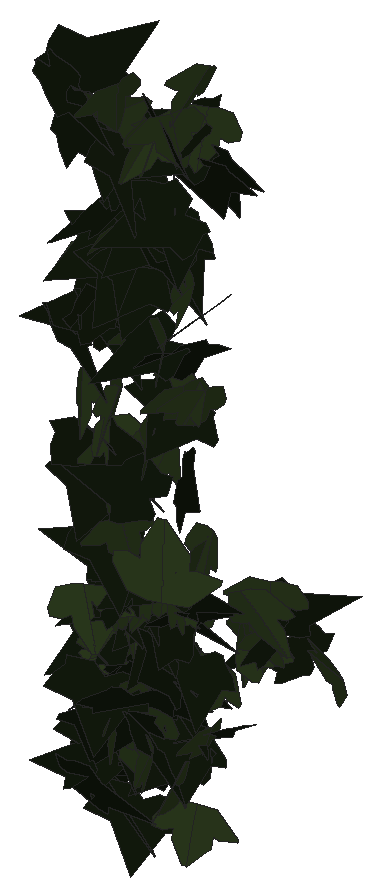
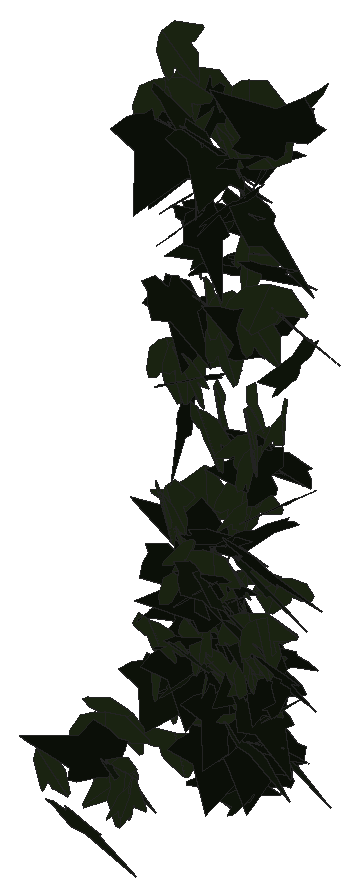
# SketchUp Ruby script. Lengths in inches.
U = 1.inch
M = Sketchup.active_model
def pt(a) = Geom::Point3d.new(a.map { |v| v * U })
def face(e, loops, mat)
  f = e.add_face(loops[0].map { |a| pt(a) })
  loops[1..].each { |l| e.add_face(l.map { |a| pt(a) }).erase! }
  f.material = f.back_material = mat if mat
  f
end
# faces: each face lists its corners as indices into pts; further lists are holes
def faces(e, pts, list, mat = nil) = list.each { |f| face(e, (f[0].is_a?(Array) ? f : [f]).map { |l| l.map { |i| pts[i] } }, mat) }
# xy, xz, yz: faces in a plane at the given z, y or x. An outline is a flat list of corners, or four numbers for a rectangle; further outlines are holes
def ring(l) = l.size == 4 ? [[l[0], l[1]], [l[2], l[1]], [l[2], l[3]], [l[0], l[3]]] : l.each_slice(2).to_a
def flat(e, list, mat, &to3) = list.each { |f| face(e, (f[0].is_a?(Array) ? f : [f]).map { |l| ring(l).map { |u, v| to3.(u, v) } }, mat) }
def xy(e, z, list, mat = nil) = flat(e, list, mat) { |x, y| [x, y, z] }
def xz(e, y, list, mat = nil) = flat(e, list, mat) { |x, z| [x, y, z] }
def yz(e, x, list, mat = nil) = flat(e, list, mat) { |y, z| [x, y, z] }
def lines(e, pts, list) = list.each { |a, b| e.add_line(pt(pts[a]), pt(pts[b])) }
# prism: a flat outline (further loops are holes) pulled along v
def prism(e, loops, v, mat = nil)
  f = face(e, loops, mat); d = Geom::Vector3d.new(v.map { |x| x * U })
  f.pushpull(f.normal.samedirection?(d) ? d.length : -d.length)
end
def box(e, o, s, mat = nil) = prism(e, [[o, [o[0] + s[0], o[1], o[2]], [o[0] + s[0], o[1] + s[1], o[2]], [o[0], o[1] + s[1], o[2]]]], [0, 0, s[2]], mat)
def at(x, y, z, deg = 0) = Geom::Transformation.translation(pt([x, y, z])) * Geom::Transformation.rotation(ORIGIN, Z_AXIS, deg.degrees)
def axes(o, x, y, z) = Geom::Transformation.new([*x, 0, *y, 0, *z, 0, *pt(o).to_a, 1])
def part(name) = M.definitions.add(name)
# library, detail: a bought-in or finely detailed component or shape, given as its bounding box
def library(name, o, s) = part(name).tap { |d| box(d.entities, o, s) }
def detail(e, o, s) = box(e.add_group.entities, o, s)
def put(e, d, t, mat = nil) = e.add_instance(d, t).tap { |i| i.material = mat if mat }
def group(e, t, mat = nil) = e.add_group.tap { |g| g.transformation = t; g.material = mat if mat }.entities
root = M.entities
M.materials.add("1026 AP 7946 SUNNY SIDE UP").color = [254, 231, 186]
M.materials.add("efeu1").color = [18, 25, 13]
M.materials.add("efeu2").color = [43, 57, 29]
c1 = part("ivyleaf_9")
p = [[1.54,2.16,1.25],[1.36,2.04,1.19],[-0.21,0.99,0.68],[-0.71,1.11,0.82],[-0.85,0.86,0.67],[-0.8,0.17,0.21],
  [-0.9,-0.01,0.1],[-0.67,-0.16,-0.02],[-0.08,-0.08,-0.05],[-0.03,-0.6,-0.4],[0.65,-0.88,-0.66],[0.83,-0.6,-0.49],
  [1.29,-0.42,-0.43],[1.8125,-0.07,-0.26],[1.21,0.44,0.15]]
faces(c1.entities,p,[[0,1,2,3,4,5,6,7,8,9,10,11,12,13,14]],"efeu1")
c2 = part("ivyleaf_10")
p = [[0,0.5,-0.03],[-0.0625,2.02,-0.43],[-0.19,2.01,-0.46],[-0.54,1.05,-0.29],[-0.52,0.625,-0.18],[-0.83,0.76,-0.28],
  [-1.16,0.64,-0.33],[-1.15,0.33,-0.24],[-0.77,-0.39,0.02],[-0.3,-0.51,0.16],[0.04,-0.48,0.23],[-0.02,2.01,-0.4375],
  [-0.06,2.01,-0.43],[0.04,-0.49,0.23],[0.67,-0.49,0.14],[1.38,0.36,-0.2],[1.375,0.51,-0.24],[0.81,0.65,-0.19],
  [0.62,0.59,-0.15],[0.6,1.09,-0.28],[0.5,1.23,-0.31]]
faces(c2.entities,p,[[0,1,2,3,4,5,6,7,8,9,10],[11,12,0,13,14,15,16,17,18,19,20]],"efeu2")
put(root,c1,axes([134.34,212.89,281.88],[-0.49432,0.03175,-0.0219],[0.02994,-0.0243,-0.32485],[-0.05228,-0.31416,0.02105]),"1026 AP 7946 SUNNY SIDE UP")
put(root,c1,axes([134.31,212.82,281.11],[-0.09783,0.301,-0.06871],[0.00789,-0.06878,-0.31692],[-0.4853,-0.0618,0.0087]),"1026 AP 7946 SUNNY SIDE UP")
put(root,c1,axes([134.45,212.35,280.29],[-0.30004,0.23825,0.08175],[-0.11148,0.04274,-0.31291],[-0.37809,-0.20166,0.02739]),"1026 AP 7946 SUNNY SIDE UP")
put(root,c1,axes([133.89,212.51,286.54],[0.25478,-0.29718,0.02731],[-0.0043,-0.03356,-0.34839],[0.46937,0.16101,-0.01802]),"1026 AP 7946 SUNNY SIDE UP")
put(root,c2,axes([134.14,212.61,285.66],[-0.04721,0.29525,-0.16134],[-0.02191,-0.15988,-0.30545],[-0.52631,-0.01983,0.02719]),"1026 AP 7946 SUNNY SIDE UP")
put(root,c2,axes([134.27,212.87,282.33],[-0.16108,-0.30575,0.02615],[0.01063,-0.03083,-0.33195],[0.48253,-0.10139,0.01604]),"1026 AP 7946 SUNNY SIDE UP")
put(root,c1,axes([133.99,212.15,290.43],[0.35,-0.27277,-0.14498],[-0.10744,0.12349,-0.36117],[0.46937,0.23167,0.02544]),"1026 AP 7946 SUNNY SIDE UP")
put(root,c1,axes([133.98,212.85,281.625],[0.43404,-0.15122,-0.01807],[-0.03969,-0.01144,-0.32351],[0.2359,0.27631,-0.02118]),"1026 AP 7946 SUNNY SIDE UP")
put(root,c1,axes([133.99,212.7,290.19],[-0.12971,-0.0235,0.37793],[0.55795,0.09367,0.08889],[-0.15183,0.3643,0.0038]),"1026 AP 7946 SUNNY SIDE UP")
put(root,c1,axes([134.66,212.68,283.28],[-0.30635,0.18692,0.20452],[-0.27383,0.10077,-0.2747],[-0.32834,-0.25845,0.03828]),"1026 AP 7946 SUNNY SIDE UP")
put(root,c1,axes([134.18,212.94,280.99],[-0.11217,-0.26826,0.15154],[0.00566,-0.15331,-0.2842],[0.48219,-0.06061,0.03859]),"1026 AP 7946 SUNNY SIDE UP")
put(root,c1,axes([134.22,212.72,284.23],[-0.16012,-0.29045,0.13158],[0.00526,-0.13681,-0.31453],[0.49994,-0.09159,0.04545]),"1026 AP 7946 SUNNY SIDE UP")
put(root,c1,axes([134.62,212.85,280.61],[-0.25845,0.26467,0.06494],[-0.07354,0.04329,-0.32025],[-0.42089,-0.17009,0.01608]),"1026 AP 7946 SUNNY SIDE UP")
put(root,c2,axes([134.37,212.9375,281.76],[-0.13891,-0.25997,0.16409],[0.04977,-0.17421,-0.27335],[0.47803,-0.0574,0.07614]),"1026 AP 7946 SUNNY SIDE UP")
put(root,c2,axes([134.45,212.86,282.375],[-0.37904,-0.20758,0.04507],[-0.03475,-0.04307,-0.32745],[0.33214,-0.2414,0.01717]),"1026 AP 7946 SUNNY SIDE UP")
put(root,c2,axes([134.28,212.73,287.6],[-0.34945,-0.2602,-0.07662],[0.22245,-0.03162,-0.32822],[0.36201,-0.23174,0.12773]),"1026 AP 7946 SUNNY SIDE UP")
put(root,c1,axes([134.74,212.23,287.14],[-0.43532,0.18322,0.08733],[-0.14006,0.0163,-0.34007],[-0.28411,-0.28878,0.03384]),"1026 AP 7946 SUNNY SIDE UP")
put(root,c1,axes([134.41,212.86,280.51],[-0.3788,-0.18587,-0.09156],[0.16254,0.00742,-0.30825],[0.27942,-0.25631,0.05518]),"1026 AP 7946 SUNNY SIDE UP")
put(root,c2,axes([134.49,212.88,281.42],[-0.2148,-0.14319,0.25708],[0.02219,-0.28001,-0.15869],[0.45296,-0.05418,0.12969]),"1026 AP 7946 SUNNY SIDE UP")
put(root,c1,axes([134.38,212,290.02],[0.20562,-0.18199,-0.30622],[-0.27433,0.23939,-0.22946],[0.47283,0.21803,0.00004]),"1026 AP 7946 SUNNY SIDE UP")
put(root,c2,axes([134.54,212.68,287.07],[-0.06667,-0.31414,0.14692],[-0.00411,-0.14519,-0.32703],[0.54363,-0.03962,0.01555]),"1026 AP 7946 SUNNY SIDE UP")
put(root,c2,axes([134.51,212.8,285.54],[0.18593,-0.30408,-0.08896],[-0.00378,0.0895,-0.33423],[0.49629,0.1146,0.03079]),"1026 AP 7946 SUNNY SIDE UP")
put(root,c1,axes([134.46,212.84,281.45],[0.45287,-0.00622,-0.2014],[-0.30741,-0.00093,-0.29675],[0.00728,0.34807,-0.00235]),"1026 AP 7946 SUNNY SIDE UP")
put(root,c2,axes([134.49,212.92,280.91],[0.32393,0.21575,-0.10349],[-0.11232,-0.07239,-0.30774],[-0.35782,0.21804,0.0029]),"1026 AP 7946 SUNNY SIDE UP")
put(root,c1,axes([134.53,212.7,280.37],[0.36929,0.14585,-0.15544],[-0.19217,-0.09055,-0.28511],[-0.26939,0.26453,-0.00969]),"1026 AP 7946 SUNNY SIDE UP")
put(root,c1,axes([134.75,212.71,287.9],[-0.48375,-0.11658,0.115],[-0.11978,-0.10852,-0.33169],[0.22458,-0.309,0.07082]),"1026 AP 7946 SUNNY SIDE UP")
put(root,c2,axes([134.55,212.67,284.85],[-0.08744,-0.32967,0.0502],[0.09737,-0.06062,-0.33707],[0.51533,-0.04449,0.07221]),"1026 AP 7946 SUNNY SIDE UP")
put(root,c1,axes([134.875,212.45,288.74],[-0.41967,0.33667,-0.1011],[0.06308,-0.09561,-0.44227],[-0.54864,-0.26852,0.02648]),"1026 AP 7946 SUNNY SIDE UP")
put(root,c2,axes([134.58,215.4375,280.83],[-0.01019,0.2895,-0.12319],[-0.03031,-0.12139,-0.29829],[-0.49257,0.00148,0.0209]),"1026 AP 7946 SUNNY SIDE UP")
put(root,c1,axes([134.25,212.72,284.79],[0.36782,-0.19375,0.14599],[0.13937,-0.11582,-0.31211],[0.35188,0.2484,-0.02899]),"1026 AP 7946 SUNNY SIDE UP")
put(root,c1,axes([134.37,212.5,285.03],[-0.22783,-0.1583,-0.28718],[0.40869,0.11944,-0.20902],[0.29297,-0.28972,0.06826]),"1026 AP 7946 SUNNY SIDE UP")
put(root,c1,axes([134.57,212.69,289.67],[-0.218,-0.32386,-0.01743],[0.01699,0.01178,-0.36282],[0.50951,-0.13896,0.00464]),"1026 AP 7946 SUNNY SIDE UP")
put(root,c2,axes([134.48,212.19,282.76],[0.44641,0.14641,0.06705],[0.11647,-0.00439,-0.32688],[-0.22281,0.29105,-0.03653]),"1026 AP 7946 SUNNY SIDE UP")
put(root,c2,axes([134.73,215.38,280.89],[-0.45718,0.11874,0.02783],[-0.06303,-0.02911,-0.32082],[-0.18056,-0.29049,0.04153]),"1026 AP 7946 SUNNY SIDE UP")
put(root,c2,axes([134.6875,212.53,288.15],[-0.06203,-0.31602,-0.14423],[0.05402,0.13482,-0.32689],[0.53966,-0.04982,0.01614]),"1026 AP 7946 SUNNY SIDE UP")
put(root,c1,axes([134.93,212.36,282.91],[-0.42089,0.17853,-0.03551],[0.02432,-0.04057,-0.3307],[-0.28518,-0.26695,0.02421]),"1026 AP 7946 SUNNY SIDE UP")
put(root,c1,axes([134.62,212.5,281.46],[0.19185,0.21668,0.20526],[0.1433,0.17588,-0.25509],[-0.43873,0.15219,0.00644]),"1026 AP 7946 SUNNY SIDE UP")
put(root,c2,axes([134.57,212.77,281.25],[0.49971,-0.03513,0.0505],[0.07043,-0.04012,-0.32769],[0.06387,0.31907,-0.03373]),"1026 AP 7946 SUNNY SIDE UP")
put(root,c1,axes([134.5,212.92,280.6],[0.06491,-0.30042,0.08418],[-0.0004,-0.08418,-0.31268],[0.49026,0.03971,-0.0114]),"1026 AP 7946 SUNNY SIDE UP")
put(root,c1,axes([134.33,212.65,281.34],[0.43737,-0.09385,0.11705],[0.1912,0.00708,-0.2992],[0.13206,0.30059,0.04553]),"1026 AP 7946 SUNNY SIDE UP")
put(root,c1,axes([134.47,212.65,286.9],[0.10754,-0.33536,-0.03255],[0.01992,0.03284,-0.35187],[0.52901,0.06694,0.01987]),"1026 AP 7946 SUNNY SIDE UP")
put(root,c2,axes([134.62,212.55,285.61],[0.29186,-0.25429,0.16201],[0.12967,-0.13614,-0.32488],[0.45314,0.20274,-0.01138]),"1026 AP 7946 SUNNY SIDE UP")
put(root,c2,axes([134.65,212.59,285.14],[0.14656,0.32508,-0.01832],[-0.03062,-0.01482,-0.34815],[-0.51117,0.09409,0.0156]),"1026 AP 7946 SUNNY SIDE UP")
put(root,c1,axes([134.31,212.27,279.96],[0.26436,-0.11381,0.24715],[0.30061,-0.14628,-0.20981],[0.29108,0.25443,-0.00779]),"1026 AP 7946 SUNNY SIDE UP")
put(root,c2,axes([134.49,212.54,289.72],[-0.40725,-0.10383,0.21891],[0.31203,0.07764,0.28791],[-0.20384,0.32628,0.00336]),"1026 AP 7946 SUNNY SIDE UP")
put(root,c1,axes([134.46,212.8,279.77],[0.23225,-0.27611,0.04535],[0.02243,-0.04405,-0.32274],[0.43946,0.14817,-0.0075]),"1026 AP 7946 SUNNY SIDE UP")
put(root,c1,axes([134.54,212.36,286.72],[-0.0681,-0.0083,0.37991],[0.47988,0.20782,0.04296],[-0.32589,0.30775,-0.01614]),"1026 AP 7946 SUNNY SIDE UP")
put(root,c2,axes([134.66,212.73,284.17],[0.0475,0.31056,-0.12657],[0.00344,-0.12531,-0.32189],[-0.52617,0.02722,-0.01353]),"1026 AP 7946 SUNNY SIDE UP")
put(root,c1,axes([134.6875,212.92,280.97],[0.27948,0.25972,0.02805],[0.05548,0.00696,-0.32314],[-0.40662,0.17946,-0.02482]),"1026 AP 7946 SUNNY SIDE UP")
put(root,c1,axes([134.67,212.47,283.64],[-0.09016,-0.32687,-0.03566],[0.03661,0.02912,-0.34122],[0.51524,-0.05927,0.01801]),"1026 AP 7946 SUNNY SIDE UP")
put(root,c1,axes([135.17,215.95,280.49],[-0.29936,0.24562,0.09847],[-0.17496,0.03017,-0.31256],[-0.37481,-0.21026,0.06725]),"1026 AP 7946 SUNNY SIDE UP")
put(root,c1,axes([134.76,212.24,281.625],[-0.35771,-0.20951,-0.1222],[0.17523,0.0512,-0.31622],[0.33454,-0.25084,0.03496]),"1026 AP 7946 SUNNY SIDE UP")
put(root,c1,axes([134.95,212.15,281.18],[0.26844,0.23427,-0.20822],[-0.15731,-0.17825,-0.29898],[-0.46183,0.19688,-0.01919]),"1026 AP 7946 SUNNY SIDE UP")
put(root,c2,axes([134.89,212.3,290.39],[-0.1518,-0.35401,-0.09394],[0.03808,0.08583,-0.37751],[0.57276,-0.09953,0.0002]),"1026 AP 7946 SUNNY SIDE UP")
put(root,c1,axes([135.1875,212.77,282.72],[-0.29015,0.26774,0.01819],[-0.04392,0.0003,-0.33416],[-0.41946,-0.18523,0.02241]),"1026 AP 7946 SUNNY SIDE UP")
put(root,c2,axes([134.88,212.34,281.11],[0.14823,-0.29081,0.08357],[0.11629,-0.06189,-0.31115],[0.46099,0.10912,0.05162]),"1026 AP 7946 SUNNY SIDE UP")
put(root,c1,axes([135.14,212.68,282.45],[-0.08693,0.31209,0.04032],[-0.02141,0.03553,-0.32622],[-0.49377,-0.05648,0.00704]),"1026 AP 7946 SUNNY SIDE UP")
put(root,c2,axes([134.66,212.95,281.42],[-0.26741,0.01935,0.2744],[0.41976,0.01239,0.17481],[-0.00009,0.31569,-0.02182]),"1026 AP 7946 SUNNY SIDE UP")
put(root,c1,axes([134.7,212.6875,282.69],[0.08552,-0.31683,-0.0483],[0.09413,0.055,-0.32344],[0.49433,0.04434,0.06995]),"1026 AP 7946 SUNNY SIDE UP")
put(root,c2,axes([135.04,212.75,286.75],[-0.08913,-0.33953,0.019],[-0.01012,-0.01958,-0.35472],[0.53474,-0.05696,-0.00354]),"1026 AP 7946 SUNNY SIDE UP")
put(root,c1,axes([135,212.81,280.21],[0.26435,0.26927,-0.02073],[-0.03264,-0.01255,-0.3269],[-0.42351,0.16904,0.01226]),"1026 AP 7946 SUNNY SIDE UP")
put(root,c2,axes([134.9,215.11,280.82],[0.07832,0.11031,0.31311],[0.0031,0.30679,-0.11348],[-0.50747,0.0189,0.04763]),"1026 AP 7946 SUNNY SIDE UP")
put(root,c2,axes([135.04,212.72,287.125],[-0.07972,-0.34126,0.04168],[0.00147,-0.04299,-0.3556],[0.54072,-0.0502,0.00711]),"1026 AP 7946 SUNNY SIDE UP")
put(root,c2,axes([134.9375,212.61,282.64],[0.04325,0.31544,-0.07608],[-0.01484,-0.0751,-0.32662],[-0.50984,0.02894,0.00305]),"1026 AP 7946 SUNNY SIDE UP")
put(root,c1,axes([134.8,212.76,288.92],[0.1524,-0.31053,-0.13178],[-0.0453,0.12312,-0.33429],[0.52508,0.10075,0.00941]),"1026 AP 7946 SUNNY SIDE UP")
put(root,c1,axes([134.73,212.89,281.67],[-0.08381,-0.03192,-0.32347],[0.49573,-0.01558,-0.05362],[-0.01588,-0.31792,0.03322]),"1026 AP 7946 SUNNY SIDE UP")
put(root,c2,axes([135.05,215.34,281.69],[-0.40877,-0.17901,0.01098],[0.03395,-0.05163,-0.32054],[0.28002,-0.25506,0.05489]),"1026 AP 7946 SUNNY SIDE UP")
put(root,c2,axes([135.02,212.28,284.01],[-0.23972,-0.29665,-0.09557],[0.10044,0.06931,-0.34228],[0.47749,-0.16351,0.02402]),"1026 AP 7946 SUNNY SIDE UP")
put(root,c1,axes([135.46,212.21,284.6],[-0.27228,0.14362,0.25167],[-0.35021,0.10651,-0.22728],[-0.27371,-0.27914,0.04046]),"1026 AP 7946 SUNNY SIDE UP")
put(root,c1,axes([134.99,212.73,279.67],[-0.31314,-0.23118,-0.09117],[0.11291,0.05299,-0.31341],[0.37172,-0.21084,0.0184]),"1026 AP 7946 SUNNY SIDE UP")
put(root,c1,axes([135.27,215.14,281.18],[-0.37695,0.21123,-0.07356],[0.06262,-0.06438,-0.32879],[-0.34558,-0.24207,0.02067]),"1026 AP 7946 SUNNY SIDE UP")
put(root,c1,axes([135.33,212.74,282.8125],[-0.08145,0.31509,-0.02285],[-0.11699,-0.03576,-0.31895],[-0.48291,-0.04448,0.08112]),"1026 AP 7946 SUNNY SIDE UP")
put(root,c2,axes([135.17,212.54,289.69],[0.30638,-0.28216,-0.11138],[-0.10068,0.08521,-0.35273],[0.46342,0.20506,-0.003]),"1026 AP 7946 SUNNY SIDE UP")
put(root,c1,axes([134.94,212.55,289.37],[-0.05308,-0.35504,0.02603],[-0.01016,-0.02679,-0.36754],[0.55982,-0.03415,-0.00421]),"1026 AP 7946 SUNNY SIDE UP")
put(root,c2,axes([135.22,212.78,283.04],[-0.46897,0.09068,0.09132],[-0.1441,0.00057,-0.32009],[-0.13701,-0.311,0.02407]),"1026 AP 7946 SUNNY SIDE UP")
put(root,c1,axes([135.31,212.82,288.5625],[0.2289,-0.00683,-0.36389],[-0.55219,0.0386,-0.14965],[0.06019,0.38006,0.01091]),"1026 AP 7946 SUNNY SIDE UP")
put(root,c2,axes([135.1875,212.57,280.74],[-0.41906,-0.20651,0.03927],[-0.02025,-0.04729,-0.3463],[0.32992,-0.26521,0.02863]),"1026 AP 7946 SUNNY SIDE UP")
put(root,c1,axes([135.1875,212.78,289.625],[0.14713,0.30954,0.1451],[-0.01553,0.1467,-0.32864],[-0.53338,0.08111,0.04959]),"1026 AP 7946 SUNNY SIDE UP")
put(root,c1,axes([135.16,212.45,287.78],[-0.36358,-0.2424,0.08279],[0.00365,-0.11217,-0.33656],[0.40222,-0.21809,0.0779]),"1026 AP 7946 SUNNY SIDE UP")
put(root,c2,axes([135.12,212.5625,282.94],[0.37813,-0.22834,0.02561],[-0.00145,-0.03881,-0.34058],[0.36139,0.23876,-0.02816]),"1026 AP 7946 SUNNY SIDE UP")
put(root,c1,axes([135.29,212.16,281.58],[0.12283,0.26206,-0.23212],[-0.09761,-0.21816,-0.28298],[-0.53615,0.09975,-0.00166]),"1026 AP 7946 SUNNY SIDE UP")
put(root,c2,axes([135.3125,212.38,281.27],[-0.46728,-0.06247,0.09837],[-0.13826,-0.04595,-0.31199],[0.11508,-0.30885,0.0246]),"1026 AP 7946 SUNNY SIDE UP")
put(root,c1,axes([135.3,212.86,282.8125],[-0.46739,-0.13291,-0.00876],[0.03059,-0.0246,-0.33412],[0.20709,-0.29633,0.02957]),"1026 AP 7946 SUNNY SIDE UP")
put(root,c2,axes([135.27,212.98,282.08],[-0.37936,0.20069,0.05525],[-0.10039,0.00477,-0.32105],[-0.31035,-0.24686,0.03632]),"1026 AP 7946 SUNNY SIDE UP")
put(root,c2,axes([135.03,214.99,281.65],[-0.40226,0.02918,-0.20537],[0.28138,-0.11568,-0.25449],[-0.14612,-0.3031,0.07531]),"1026 AP 7946 SUNNY SIDE UP")
put(root,c2,axes([135.23,212.56,283.04],[0.40473,-0.20996,0.02381],[0.00403,-0.0352,-0.34139],[0.33233,0.25614,-0.02486]),"1026 AP 7946 SUNNY SIDE UP")
put(root,c1,axes([135.21,212.53,287.77],[-0.21547,-0.31459,0.07296],[-0.01957,-0.07367,-0.35346],[0.50728,-0.13646,0.01736]),"1026 AP 7946 SUNNY SIDE UP")
put(root,c1,axes([134.98,215.49,281.24],[0.06415,0.055,0.31824],[0.47036,0.08618,-0.05606],[-0.14731,0.29912,-0.04041]),"1026 AP 7946 SUNNY SIDE UP")
put(root,c1,axes([135.59,212.95,281.67],[-0.44457,0.14638,0.01165],[-0.08144,-0.07824,-0.31407],[-0.21591,-0.27189,0.09447]),"1026 AP 7946 SUNNY SIDE UP")
put(root,c2,axes([135.27,212.4,281.7],[-0.21207,-0.24351,-0.16211],[0.14953,0.12519,-0.28533],[0.42943,-0.16385,0.01929]),"1026 AP 7946 SUNNY SIDE UP")
put(root,c2,axes([135.19,213,281.4],[-0.09372,0.12118,-0.29457],[0.1151,-0.27818,-0.13847],[-0.47558,-0.09121,0.02453]),"1026 AP 7946 SUNNY SIDE UP")
put(root,c1,axes([135.55,212.68,283.33],[-0.46188,-0.11083,0.09058],[-0.11403,-0.05769,-0.32255],[0.19172,-0.30133,0.02637]),"1026 AP 7946 SUNNY SIDE UP")
put(root,c1,axes([135.49,212.63,288.5],[-0.47818,-0.16707,0.04463],[-0.03904,-0.04644,-0.35652],[0.26894,-0.30379,0.0276]),"1026 AP 7946 SUNNY SIDE UP")
put(root,c1,axes([135.46,212.42,281.75],[0.37419,0.11505,-0.26129],[-0.34188,-0.1331,-0.27244],[-0.27516,0.32183,-0.01682]),"1026 AP 7946 SUNNY SIDE UP")
put(root,c1,axes([135.39,212.9,281.49],[0.3612,0.18189,-0.13009],[-0.15173,-0.08318,-0.3023],[-0.31441,0.24911,-0.00356]),"1026 AP 7946 SUNNY SIDE UP")
put(root,c1,axes([135.21,212.84,282.72],[0.00683,-0.32586,0.01145],[0.01609,-0.01283,-0.33564],[0.51253,0.00474,0.01039]),"1026 AP 7946 SUNNY SIDE UP")
put(root,c2,axes([135.46,212.37,289.9],[0.14242,0.26653,-0.2121],[-0.1924,-0.17424,-0.28675],[-0.49495,0.14442,0.05043]),"1026 AP 7946 SUNNY SIDE UP")
put(root,c1,axes([135.02,212.95,282.63],[0.42561,-0.09394,0.14398],[0.20411,-0.05372,-0.29538],[0.16977,0.3001,-0.00583]),"1026 AP 7946 SUNNY SIDE UP")
put(root,c1,axes([135.67,212.98,281.6875],[-0.39161,-0.07981,0.18667],[-0.23998,-0.10924,-0.26564],[0.19937,-0.28826,0.04693]),"1026 AP 7946 SUNNY SIDE UP")
put(root,c1,axes([135.65,212.4,286.89],[-0.52945,0.06122,-0.04568],[0.0423,-0.09372,-0.34163],[-0.11143,-0.32649,0.08736]),"1026 AP 7946 SUNNY SIDE UP")
put(root,c2,axes([135.42,212.34,285.41],[0.2414,-0.30014,-0.0532],[0.02415,0.06351,-0.34421],[0.47781,0.14843,0.04427]),"1026 AP 7946 SUNNY SIDE UP")
put(root,c2,axes([135.45,212.6,285.17],[0.42946,-0.19364,-0.0614],[-0.04685,0.05872,-0.34316],[0.31461,0.27308,0.03272]),"1026 AP 7946 SUNNY SIDE UP")
put(root,c1,axes([135.66,212.85,280.7],[-0.49265,-0.05089,-0.02868],[0.05099,-0.02876,-0.32535],[0.07536,-0.3132,0.03264]),"1026 AP 7946 SUNNY SIDE UP")
put(root,c2,axes([135.55,212.12,280.84],[0.2566,-0.27588,-0.10951],[-0.04649,0.10379,-0.32851],[0.46166,0.16379,0.02778]),"1026 AP 7946 SUNNY SIDE UP")
put(root,c1,axes([135.78,212.8,289.74],[-0.55419,0.03512,0.01297],[-0.0248,-0.03396,-0.36327],[-0.05305,-0.35103,0.03434]),"1026 AP 7946 SUNNY SIDE UP")
put(root,c2,axes([135.59,212.84,282.66],[-0.3034,-0.25068,0.04706],[0.01546,-0.06633,-0.32255],[0.40076,-0.18721,0.04807]),"1026 AP 7946 SUNNY SIDE UP")
put(root,c1,axes([135.24,212.61,288.15],[0.31302,-0.29419,0.01357],[0.01918,-0.00966,-0.36596],[0.46277,0.19939,0.006]),"1026 AP 7946 SUNNY SIDE UP")
put(root,c1,axes([135.32,213.09,281.38],[0.10212,-0.30688,0.04347],[0.04509,-0.03875,-0.32273],[0.48538,0.06817,0.02084]),"1026 AP 7946 SUNNY SIDE UP")
put(root,c1,axes([135.65,212.53,282.57],[-0.46623,-0.01327,-0.14181],[0.21562,-0.06902,-0.298],[-0.02722,-0.3195,0.06831]),"1026 AP 7946 SUNNY SIDE UP")
put(root,c1,axes([135.61,212.29,290.19],[0.38848,-0.08063,-0.28514],[-0.41771,0.07636,-0.2672],[0.17429,0.36272,-0.00481]),"1026 AP 7946 SUNNY SIDE UP")
put(root,c1,axes([135.33,212.36,281.0625],[0.24606,-0.29251,0.01158],[-0.01212,-0.01874,-0.34149],[0.46024,0.1559,-0.01518]),"1026 AP 7946 SUNNY SIDE UP")
put(root,c1,axes([135.77,212.43,288.95],[0.13774,-0.08152,-0.37715],[-0.5109,0.17037,-0.11832],[0.29319,0.33517,-0.029]),"1026 AP 7946 SUNNY SIDE UP")
put(root,c2,axes([135.6875,212.23,286.95],[0.25331,-0.28481,-0.16756],[-0.03972,0.16813,-0.33139],[0.51293,0.15367,0.05709]),"1026 AP 7946 SUNNY SIDE UP")
put(root,c1,axes([135.68,212.77,285.8],[-0.31005,-0.25152,0.11931],[0.00774,-0.14698,-0.31716],[0.43628,-0.17614,0.09042]),"1026 AP 7946 SUNNY SIDE UP")
put(root,c1,axes([135.9,212.83,287.17],[-0.16604,0.31595,-0.08137],[0.01359,-0.08217,-0.3432],[-0.5126,-0.10452,0.01726]),"1026 AP 7946 SUNNY SIDE UP")
put(root,c1,axes([136.01,212.26,288.96],[-0.53778,-0.02428,0.07538],[-0.10862,-0.05265,-0.35026],[0.05429,-0.34579,0.04595]),"1026 AP 7946 SUNNY SIDE UP")
put(root,c1,axes([135.87,212.62,282.82],[0.09532,0.30441,-0.087],[-0.06971,-0.07871,-0.319],[-0.49256,0.07005,0.02831]),"1026 AP 7946 SUNNY SIDE UP")
put(root,c1,axes([135.69,212.4,282.03],[-0.1419,-0.09891,0.31175],[-0.07673,-0.30709,-0.11997],[0.49554,-0.07587,0.0707]),"1026 AP 7946 SUNNY SIDE UP")
put(root,c2,axes([135.79,212.71,286.08],[0.40425,-0.21829,-0.03928],[-0.06016,0.01187,-0.34701],[0.34287,0.25945,-0.01457]),"1026 AP 7946 SUNNY SIDE UP")
put(root,c1,axes([135.57,212.77,288.37],[0.07549,-0.34639,0.01503],[0.00004,-0.01671,-0.36035],[0.54529,0.04795,-0.00205]),"1026 AP 7946 SUNNY SIDE UP")
put(root,c2,axes([135.81,212.54,286.12],[-0.19549,-0.32224,-0.05795],[0.04899,0.04628,-0.35532],[0.51152,-0.12758,0.01188]),"1026 AP 7946 SUNNY SIDE UP")
put(root,c1,axes([136.05,212.6875,290.15],[-0.37828,0.25147,-0.06275],[0.0457,-0.05834,-0.35833],[-0.40481,-0.24157,0.01818]),"1026 AP 7946 SUNNY SIDE UP")
put(root,c2,axes([135.75,212.57,283.06],[0.00851,0.32685,0.03078],[-0.02533,0.02825,-0.33617],[-0.5152,0.00401,0.01704]),"1026 AP 7946 SUNNY SIDE UP")
put(root,c1,axes([135.84,212.31,286.8125],[0.21777,0.31915,-0.00267],[0.02051,-0.01046,-0.35809],[-0.50147,0.13817,-0.0158]),"1026 AP 7946 SUNNY SIDE UP")
put(root,c1,axes([135.67,212.62,288.71],[-0.0522,-0.33954,0.10545],[0.00609,-0.10508,-0.3518],[0.55848,-0.03059,0.0137]),"1026 AP 7946 SUNNY SIDE UP")
put(root,c1,axes([135.74,212.78,280.91],[-0.14345,-0.30436,0.01667],[0.02145,-0.02275,-0.32684],[0.47892,-0.09015,0.01963]),"1026 AP 7946 SUNNY SIDE UP")
put(root,c2,axes([135.81,212.11,283.46],[0.57138,0.17272,-0.02037],[-0.00197,0.05065,0.41204],[0.27352,-0.36043,0.04551]),"1026 AP 7946 SUNNY SIDE UP")
put(root,c2,axes([136.08,215.34,280.81],[0.17122,-0.00166,-0.31754],[-0.2784,0.26724,-0.06436],[0.39671,0.18826,0.09188]),"1026 AP 7946 SUNNY SIDE UP")
put(root,c2,axes([135.86,212.28,290.27],[-0.28135,-0.31007,-0.0777],[0.10981,0.04427,-0.36651],[0.48894,-0.18836,0.03761]),"1026 AP 7946 SUNNY SIDE UP")
put(root,c1,axes([135.92,212.8,280.94],[0.25294,0.25714,0.11044],[0.00396,0.12081,-0.3059],[-0.43717,0.14988,0.06113]),"1026 AP 7946 SUNNY SIDE UP")
put(root,c1,axes([135.5,212.53,283.17],[0.18242,-0.06668,0.30772],[0.37466,-0.18145,-0.13795],[0.30295,0.26454,-0.01469]),"1026 AP 7946 SUNNY SIDE UP")
put(root,c1,axes([135.8125,212.86,289.63],[0.60055,0.04179,-0.15199],[-0.22479,-0.0479,-0.39489],[-0.08818,0.40671,-0.02845]),"1026 AP 7946 SUNNY SIDE UP")
put(root,c2,axes([135.97,212.7,283.79],[0.06945,-0.33218,0.00265],[0.01313,-0.00338,-0.34515],[0.52221,0.04426,0.00833]),"1026 AP 7946 SUNNY SIDE UP")
put(root,c1,axes([136.04,212.28,285.05],[0.12731,-0.10651,-0.35703],[-0.42492,0.21808,-0.13304],[0.37869,0.28051,-0.02926]),"1026 AP 7946 SUNNY SIDE UP")
put(root,c2,axes([136.03,212.65,286.08],[-0.20191,-0.31677,0.01874],[-0.00183,-0.0211,-0.35218],[0.49907,-0.12823,0.00629]),"1026 AP 7946 SUNNY SIDE UP")
put(root,c2,axes([135.87,212.14,280.18],[0.06862,-0.34401,0.01832],[0.01859,0.02138,0.35705],[-0.54149,-0.04286,0.01458]),"1026 AP 7946 SUNNY SIDE UP")
put(root,c1,axes([135.9,212.66,289.49],[0.48497,0.1232,-0.11821],[-0.15491,-0.06391,-0.3418],[-0.21559,0.32306,-0.0203]),"1026 AP 7946 SUNNY SIDE UP")
put(root,c2,axes([136.03,212.79,281.02],[-0.02675,-0.32104,-0.00933],[0.00144,0.00719,-0.33116],[0.50493,-0.01703,0.00045]),"1026 AP 7946 SUNNY SIDE UP")
put(root,c2,axes([136.12,212.22,287.94],[0.20419,-0.26477,-0.21049],[-0.14499,0.18067,-0.30273],[0.504,0.15924,-0.00181]),"1026 AP 7946 SUNNY SIDE UP")
put(root,c2,axes([136,213.01,281.83],[0.45963,-0.12128,-0.03618],[-0.04162,0.02596,-0.32557],[0.19381,0.29318,0.01589]),"1026 AP 7946 SUNNY SIDE UP")
put(root,c2,axes([135.96,212.86,283.82],[0.36612,-0.2288,0.04757],[0.07867,-0.01665,-0.33556],[0.3589,0.23705,0.02503]),"1026 AP 7946 SUNNY SIDE UP")
put(root,c2,axes([136.07,212.69,290.22],[-0.38109,-0.25786,0.06305],[0.05913,-0.11739,-0.34846],[0.41304,-0.2211,0.10806]),"1026 AP 7946 SUNNY SIDE UP")
put(root,c2,axes([136.09,212.55,290.92],[-0.01597,-0.31984,0.1682],[0.01074,-0.16529,-0.33045],[0.56586,-0.00589,0.01102]),"1026 AP 7946 SUNNY SIDE UP")
put(root,c1,axes([135.95,212.75,282.13],[-0.12315,-0.30848,0.01876],[0.00262,-0.02101,-0.32792],[0.48606,-0.07805,0.00652]),"1026 AP 7946 SUNNY SIDE UP")
put(root,c2,axes([135.99,212.55,279.89],[0.46906,0.11024,-0.01555],[-0.0162,-0.01745,-0.32746],[-0.17434,0.29821,-0.01142]),"1026 AP 7946 SUNNY SIDE UP")
